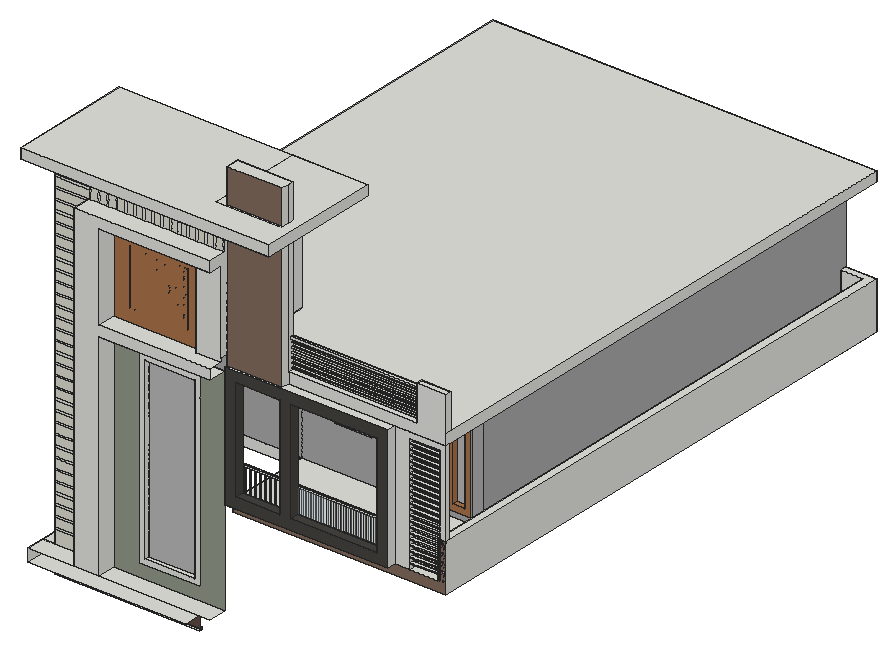
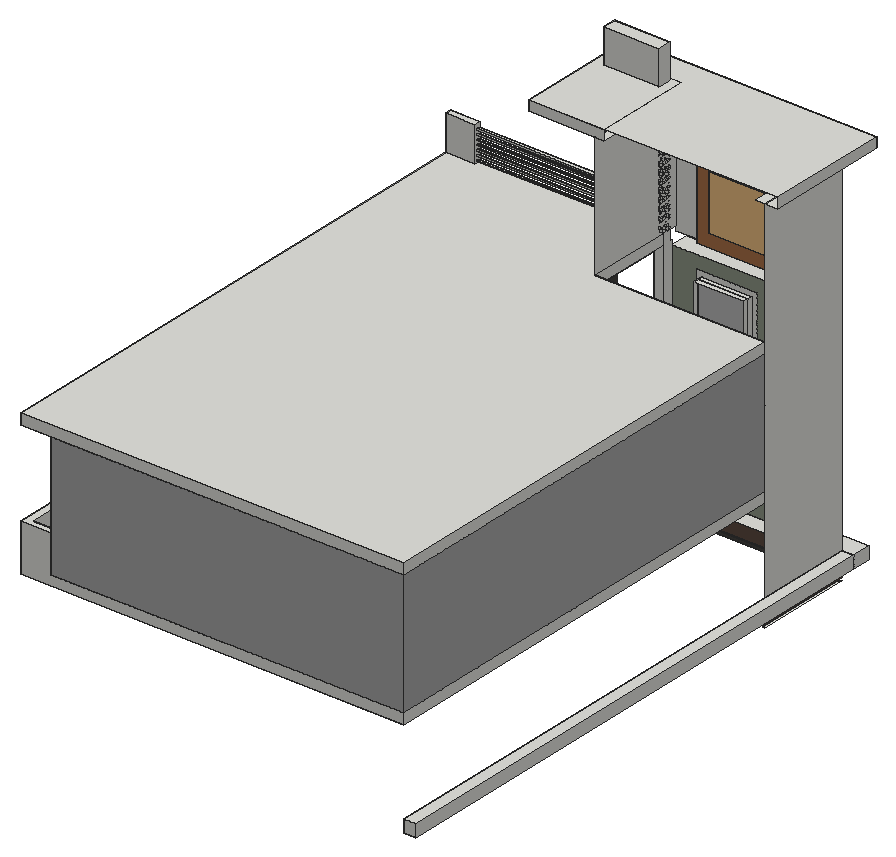
# SketchUp Ruby script. Lengths in inches.
U = 1.inch
M = Sketchup.active_model
def pt(a) = Geom::Point3d.new(a.map { |v| v * U })
def face(e, loops, mat)
  f = e.add_face(loops[0].map { |a| pt(a) })
  loops[1..].each { |l| e.add_face(l.map { |a| pt(a) }).erase! }
  f.material = f.back_material = mat if mat
  f
end
# faces: each face lists its corners as indices into pts; further lists are holes
def faces(e, pts, list, mat = nil) = list.each { |f| face(e, (f[0].is_a?(Array) ? f : [f]).map { |l| l.map { |i| pts[i] } }, mat) }
# xy, xz, yz: faces in a plane at the given z, y or x. An outline is a flat list of corners, or four numbers for a rectangle; further outlines are holes
def ring(l) = l.size == 4 ? [[l[0], l[1]], [l[2], l[1]], [l[2], l[3]], [l[0], l[3]]] : l.each_slice(2).to_a
def flat(e, list, mat, &to3) = list.each { |f| face(e, (f[0].is_a?(Array) ? f : [f]).map { |l| ring(l).map { |u, v| to3.(u, v) } }, mat) }
def xy(e, z, list, mat = nil) = flat(e, list, mat) { |x, y| [x, y, z] }
def xz(e, y, list, mat = nil) = flat(e, list, mat) { |x, z| [x, y, z] }
def yz(e, x, list, mat = nil) = flat(e, list, mat) { |y, z| [x, y, z] }
def lines(e, pts, list) = list.each { |a, b| e.add_line(pt(pts[a]), pt(pts[b])) }
# prism: a flat outline (further loops are holes) pulled along v
def prism(e, loops, v, mat = nil)
  f = face(e, loops, mat); d = Geom::Vector3d.new(v.map { |x| x * U })
  f.pushpull(f.normal.samedirection?(d) ? d.length : -d.length)
end
def box(e, o, s, mat = nil) = prism(e, [[o, [o[0] + s[0], o[1], o[2]], [o[0] + s[0], o[1] + s[1], o[2]], [o[0], o[1] + s[1], o[2]]]], [0, 0, s[2]], mat)
def at(x, y, z, deg = 0) = Geom::Transformation.translation(pt([x, y, z])) * Geom::Transformation.rotation(ORIGIN, Z_AXIS, deg.degrees)
def axes(o, x, y, z) = Geom::Transformation.new([*x, 0, *y, 0, *z, 0, *pt(o).to_a, 1])
def part(name) = M.definitions.add(name)
# library, detail: a bought-in or finely detailed component or shape, given as its bounding box
def library(name, o, s) = part(name).tap { |d| box(d.entities, o, s) }
def detail(e, o, s) = box(e.add_group.entities, o, s)
def put(e, d, t, mat = nil) = e.add_instance(d, t).tap { |i| i.material = mat if mat }
def group(e, t, mat = nil) = e.add_group.tap { |g| g.transformation = t; g.material = mat if mat }.entities
root = M.entities
M.materials.add("Glass_Mirror_01").color = [185, 185, 185]
M.materials.add("Glass_Safety_01").color = [2, 2, 2]
M.materials["Glass_Safety_01"].alpha = 0.62
M.materials.add("Glass_Safety_1").color = [204, 235, 244]
M.materials["Glass_Safety_1"].alpha = 0.25
M.materials.add("Image5").color = [194, 200, 205]
M.materials.add("Image7").color = [145, 153, 137]
M.materials.add("M03_Pewter_Shine").color = [168, 168, 168]
M.materials.add("Metal_06_1K").color = [238, 236, 231]
M.materials.add("Milk_White_Licetto-washable_matte_wall_paint").color = [220, 220, 208]
M.materials.add("Wood_Floor_12_1K").color = [132, 108, 93]
M.materials.add("Wood_Floor_12_1K1").color = [92, 75, 65]
M.materials.add("Wood_Planks_01_1K").color = [69, 67, 63]
M.materials.add("Wood_Veneer_15_1K").color = [170, 114, 74]
c1 = library("ganesh ",[0,0,0],[14.78,0.5,14.79])
xy(root,142.01,[[12,57.125,153,59.125],[12,59.125,14,150.125]])
xy(root,144.01,[[12,57.125,153,59.125],[12,59.125,14,150.125]])
xy(root,156.01,[[0,39.125,153,57.125],[0,57.125,12,588.125]])
xy(root,168.01,[[0,39.125,45,57.125],[69,39.125,177,57.125],[0,57.125,12,588.125]])
xy(root,185.46,[[99.34,57.125,147.79,61.625],[99.34,61.625,147.79,66.125]])
xy(root,292.18,[[226.96,67.38,227.77,67.96]])
xy(root,358.09,[[99.34,57.125,147.79,61.625],[99.34,61.625,147.79,66.125]])
xy(root,376,[[69,39.125,177,57.125]])
xy(root,386,[[69,39.125,177,39.125,177,52.125,153,52.125,153,57.125,69,57.125]])
xy(root,469.49,[[69,39.125,69,57.125,153,57.125,153,52.125,177,52.125,177,39.125]])
xy(root,479.49,[[45,39.125,177,57.125]])
xy(root,510,[[0,30.125,0,57.125,177,57.125,177,150.125,241.26,150.125,241.26,30.125],[0,57.125,12,66.125],[12,57.125,168,66.125],[168,57.125,175,150.125],[175,57.125,177,150.125],
  [0,66.125,12,150.125],[12,66.125,21,150.125]])
xy(root,520,[[0,30.125,241.26,150.125]])
xz(root,30.125,[[0,510,241.26,520]])
xz(root,39.125,[[45,168.01,69,168.01,69,376,177,376,177,386,69,386,69,469.49,177,469.49,177,479.49,45,479.49]])
xz(root,52.125,[[153,386,177,469.49]])
xz(root,57.125,[[0,156.01,12,168.01],[[94.34,180.46,152.79,363.09],[99.34,185.46,147.79,358.09]],[12,181.04,45,183.04],[12,191.26,45,193.26],[12,201.47,45,203.47],
  [12,211.68,45,213.68],[12,221.89,45,223.89],[12,232.1,45,234.1],[12,242.32,45,244.32],[12,252.53,45,254.53],
  [12,262.74,45,264.74],[12,272.95,45,274.95],[12,283.16,45,285.16],[12,293.375,45,295.375],[12,303.59,45,305.59],
  [12,313.8,45,315.8],[12,324.01,45,326.01],[12,334.22,45,336.22],[12,344.4375,45,346.4375],[12,354.65,45,356.65],
  [12,364.86,45,366.86],[12,375.07,45,377.07],[12,385.28,45,387.28],[12,395.5,45,397.5],[12,405.71,45,407.71],
  [12,415.92,45,417.92],[12,426.13,45,428.13],[12,436.34,45,438.34],[12,446.56,45,448.56],[12,456.77,45,458.77],
  [12,466.98,45,468.98],[12,477.19,45,479.19],[45,479.49,47,510],[53.67,479.49,55.67,510],[62.33,479.49,64.34,510],
  [71,479.49,73,510],[79.67,479.49,81.67,510],[88.33,479.49,90.34,510],[97,479.49,99,510],[105.66,479.49,107.67,510],
  [114.33,479.49,116.34,510],[123,479.49,125,510],[131.66,479.49,133.67,510],[140.33,479.49,142.33,510],[149,479.49,151,510],
  [157.66,479.49,159.67,510],[166.33,479.49,168.33,510],[175,479.49,177,510],[12,487.4,45,489.4]])
xz(root,57.125,[[[69,168.01,177,376],[94.34,180.46,152.79,363.09]]],"Image7")
xz(root,57.125,[[12,168.01,45,181.04],[12,183.04,45,191.26],[12,193.26,45,201.47],[12,203.47,45,211.68],[12,213.68,45,221.89],
  [12,223.89,45,232.1],[12,234.1,45,242.32],[12,244.32,45,252.53],[12,254.53,45,262.74],[12,264.74,45,272.95],
  [12,274.95,45,283.16],[12,285.16,45,293.375],[12,295.375,45,303.59],[12,305.59,45,313.8],[12,315.8,45,324.01],
  [12,326.01,45,334.22],[12,336.22,45,344.4375],[12,346.4375,45,354.65],[12,356.65,45,364.86],[12,366.86,45,375.07],
  [12,377.07,45,385.28],[12,387.28,45,395.5],[12,397.5,45,405.71],[12,407.71,45,415.92],[12,417.92,45,426.13],
  [12,428.13,45,436.34],[12,438.34,45,446.56],[12,448.56,45,456.77],[12,458.77,45,466.98],[12,468.98,45,477.19],
  [12,479.19,45,487.4],[47,479.49,53.67,510],[55.67,479.49,62.33,510],[64.34,479.49,71,510],[73,479.49,79.67,510],
  [81.67,479.49,88.33,510],[90.34,479.49,97,510],[99,479.49,105.66,510],[107.67,479.49,114.33,510],[116.34,479.49,123,510],
  [125,479.49,131.66,510],[133.67,479.49,140.33,510],[142.33,479.49,149,510],[151,479.49,157.66,510],[159.67,479.49,166.33,510],
  [168.33,479.49,175,510],[12,489.4,45,510]],"Milk_White_Licetto-washable_matte_wall_paint")
xz(root,57.125,[[12,144.01,153,156.01]],"Wood_Floor_12_1K1")
xz(root,57.125,[[69,386,153,469.49]],"Wood_Veneer_15_1K")
xz(root,59.125,[[14,142.01,153,144.01]],"Wood_Planks_01_1K")
xz(root,61.625,[[99.34,185.46,147.79,358.09]],"Glass_Mirror_01")
xz(root,67.77,[[243.15,266.81,243.85,292.18],[246.4,266.81,247.1,292.18],[249.64,266.81,250.34,292.18],[252.89,266.81,253.59,292.18],[256.13,266.81,256.83,292.18],
  [259.38,266.81,260.08,292.18],[262.625,266.81,263.32,292.18],[267.49,266.81,268.19,292.18],[270.74,266.81,271.4375,292.18],[273.98,266.81,274.68,292.18],
  [277.23,266.81,277.93,292.18],[280.47,266.81,281.17,292.18],[283.72,266.81,284.42,292.18],[286.96,266.81,287.66,292.18],[290.21,266.81,290.91,292.18],
  [293.45,266.81,294.15,292.18],[296.7,266.81,297.4,292.18],[299.94,266.81,300.64,292.18],[303.1875,266.81,303.89,292.18],[306.43,266.81,307.13,292.18],
  [309.68,266.81,310.38,292.18],[312.92,266.81,313.62,292.18],[316.17,266.81,316.87,292.18],[319.41,266.81,320.11,292.18],[322.66,266.81,323.36,292.18]])
xz(root,67.77,[[240.53,266.81,240.61,292.18]],"Glass_Safety_1")
xz(root,150.125,[[168,510,241.26,520]])
xz(root,588.125,[[0,156.01,12,168.01]])
yz(root,0,[[39.125,156.01,57.125,168.01],[57.125,156.01,588.125,168.01],[30.125,510,150.125,520]])
yz(root,12,[[57.125,156.01,150.125,168.01],[150.125,156.01,588.125,168.01],[57.125,168.01,150.125,510]])
yz(root,12,[[57.125,144.01,150.125,156.01]],"Wood_Floor_12_1K1")
yz(root,14,[[59.125,142.01,150.125,144.01]],"Wood_Planks_01_1K")
yz(root,45,[[39.125,168.01,57.125,479.49]])
yz(root,69,[[39.125,168.01,57.125,376],[39.125,386,57.125,469.49]])
yz(root,99.34,[[57.125,185.46,61.625,358.09],[61.625,185.46,66.125,358.09]])
yz(root,147.79,[[57.125,185.46,61.625,358.09],[61.625,185.46,66.125,358.09]])
yz(root,153,[[52.125,386,57.125,469.49]])
yz(root,177,[[52.125,390,150.125,390,150.125,510,57.125,510,57.125,479.49,39.125,479.49,39.125,469.49,52.125,469.49]])
yz(root,241.26,[[30.125,510,150.125,520]])
p = [[334.61,67.85,292.18],[243.85,67.77,292.18],[243.85,67.77,266.81],[243.23,67.77,266.81],[243.15,67.77,266.81],[243.15,67.77,292.18],
  [240.61,67.77,292.18],[240.61,67.77,266.81],[240.53,67.77,266.81],[240.53,67.77,292.18],[240.32,67.77,292.18],[233.65,67.77,292.18],
  [233.65,67.77,262.23],[334.61,67.85,262.23],[240.32,67.77,269.07],[240.32,67.77,266.81],[244.85,67.77,266.81],[245.48,67.77,266.81],
  [245.48,67.77,292.18],[244.78,67.77,292.18],[244.78,67.77,266.81],[248.1,67.77,266.81],[248.72,67.77,266.81],[248.72,67.77,292.18],
  [248.02,67.77,292.18],[248.02,67.77,266.81],[251.34,67.77,266.81],[251.97,67.77,266.81],[251.97,67.77,292.18],[251.27,67.77,292.18],
  [251.27,67.77,266.81],[254.59,67.77,266.81],[255.21,67.77,266.81],[255.21,67.77,292.18],[254.51,67.77,292.18],[254.51,67.77,266.81],
  [257.83,67.77,266.81],[258.46,67.77,266.81],[258.46,67.77,292.18],[257.76,67.77,292.18],[257.76,67.77,266.81],[261.08,67.77,266.81],
  [261.7,67.77,266.81],[261.7,67.77,292.18],[261,67.77,292.18],[261,67.77,266.81],[264.32,67.77,266.81],[264.95,67.77,266.81],
  [264.95,67.77,292.18],[264.25,67.77,292.18],[264.25,67.77,266.81],[265.95,67.77,266.81],[266.57,67.77,266.81],[266.57,67.77,292.18],
  [265.87,67.77,292.18],[265.87,67.77,266.81],[269.19,67.77,266.81],[269.8125,67.77,266.81],[269.8125,67.77,292.18],[269.11,67.77,292.18],
  [269.11,67.77,266.81],[272.4375,67.77,266.81],[273.06,67.77,266.81],[273.06,67.77,292.18],[272.36,67.77,292.18],[272.36,67.77,266.81],
  [275.68,67.77,266.81],[276.3,67.77,266.81],[276.3,67.77,292.18],[275.6,67.77,292.18],[275.6,67.77,266.81],[278.93,67.77,266.81],
  [279.55,67.77,266.81],[279.55,67.77,292.18],[278.85,67.77,292.18],[278.85,67.77,266.81],[282.17,67.77,266.81],[282.79,67.77,266.81],
  [282.79,67.77,292.18],[282.09,67.77,292.18],[282.09,67.77,266.81],[285.42,67.77,266.81],[286.04,67.77,266.81],[286.04,67.77,292.18],
  [285.34,67.77,292.18],[285.34,67.77,266.81],[288.66,67.77,266.81],[289.28,67.77,266.81],[289.28,67.77,292.18],[288.58,67.77,292.18],
  [288.58,67.77,266.81],[291.91,67.77,266.81],[292.53,67.77,266.81],[292.53,67.77,292.18],[291.83,67.77,292.18],[291.83,67.77,266.81],
  [295.15,67.77,266.81],[295.77,67.77,266.81],[295.77,67.77,292.18],[295.07,67.77,292.18],[295.07,67.77,266.81],[298.4,67.77,266.81],
  [299.02,67.77,266.81],[299.02,67.77,292.18],[298.32,67.77,292.18],[298.32,67.77,266.81],[168,57.125,520],[230.05,57.125,520],
  [229.85,72.13,519.8],[230.05,72.13,510],[168,150.125,520]]
faces(root,p,[[0,1,2,3,4,5,6,7,8,9,10,11,12,13]],"Glass_Safety_1")
lines(root,p,[[10,14],[14,15],[16,17],[18,19],[20,16],[21,22],[23,24],[25,21],[26,27],[28,29],[30,26],[31,32],
  [33,34],[35,31],[36,37],[38,39],[40,36],[41,42],[43,44],[45,41],[46,47],[48,49],[50,46],[51,52],
  [53,54],[55,51],[56,57],[58,59],[60,56],[61,62],[63,64],[65,61],[66,67],[68,69],[70,66],[71,72],
  [73,74],[75,71],[76,77],[78,79],[80,76],[81,82],[83,84],[85,81],[86,87],[88,89],[90,86],[91,92],
  [93,94],[95,91],[96,97],[98,99],[100,96],[101,102],[103,104],[105,101],[106,107],[108,109],[106,110]])
g1 = group(root,at(12,150.125,250))
xy(g1,0,[[165,-84,165,0,0,0,0,438,372,438,372,-84]])
xy(g1,10,[[165,-84,363.98,-84,363.98,431.93,342,431.93,342,438,0,438,0,0,165,0]])
xy(g1,46,[[363.98,-84,372,-84,372,438,342,438,342,431.93,363.98,431.93]])
xz(g1,-84,[[165,0,372,0,372,46,363.98,46,363.98,10,165,10]],"Wood_Floor_12_1K")
xz(g1,0,[[0,0,165,10]])
xz(g1,431.93,[[342,10,363.98,46]])
xz(g1,438,[[0,0,0,10,342,10,342,46,372,46,372,0]])
yz(g1,0,[[0,0,438,10]])
yz(g1,165,[[-84,0,0,10]])
yz(g1,342,[[431.93,10,438,46]])
yz(g1,363.98,[[-84,10,431.93,46]])
yz(g1,372,[[-84,0,438,46]])
g2 = group(root,at(12,150.125,260),"M03_Pewter_Shine")
xy(g2,0,[[9,9,333,429]])
xy(g2,6,[[258,-1,330,0]])
xy(g2,12,[[264,4.5,276,9],[281,4.5,307,9],[312,4.5,324,9]])
xy(g2,12,[[264,-1,276,4.5],[281,-1,307,4.5],[312,-1,324,4.5]],"Wood_Veneer_15_1K")
xy(g2,42,[[198,-1,234,0]])
xy(g2,45,[[201,4.5,214.5,9],[217.5,4.5,231,9]])
xy(g2,45,[[201,-1,214.5,4.5],[217.5,-1,231,4.5]],"Wood_Planks_01_1K")
xy(g2,87,[[201,4.5,214.5,9],[217.5,4.5,231,9]])
xy(g2,87,[[201,-1,214.5,4.5],[217.5,-1,231,4.5]],"Wood_Planks_01_1K")
xy(g2,90,[[198,-1,234,0],[264,4.5,276,9],[281,4.5,307,9],[312,4.5,324,9]])
xy(g2,90,[[264,-1,276,4.5],[281,-1,307,4.5],[312,-1,324,4.5]],"Wood_Veneer_15_1K")
xy(g2,96,[[258,-1,330,0]])
xy(g2,120,[[[0,0,342,438],[9,9,333,429]]])
xz(g2,-1,[[[198,42,234,90],[199.48,43.48,232.52,88.52]]])
xz(g2,-1,[[[199.48,43.48,232.52,88.52],[201,45,214.5,87],[217.5,45,231,87]]],"Wood_Planks_01_1K")
xz(g2,-1,[[[258,6,330,96],[281,12,307,90],[264,12,276,90],[312,12,324,90]]],"Wood_Veneer_15_1K")
xz(g2,0,[[0,0,9,120],[9,0,156,120],[156,0,165,120],[[165,0,342,120],[258,6,330,96],[198,42,234,90]]])
xz(g2,4.5,[[264,12,276,90],[281,12,307,90],[312,12,324,90]],"Glass_Mirror_01")
xz(g2,4.5,[[201,45,214.5,87],[217.5,45,231,87]],"Glass_Safety_01")
xz(g2,9,[[[9,0,333,120],[281,12,307,90],[264,12,276,90],[312,12,324,90],[201,45,214.5,87],[217.5,45,231,87]]])
xz(g2,429,[[9,0,333,120]])
xz(g2,438,[[0,0,342,120]])
yz(g2,0,[[0,0,438,120]])
yz(g2,9,[[9,0,429,120]])
yz(g2,198,[[-1,42,0,90]])
yz(g2,201,[[4.5,45,9,87]])
yz(g2,201,[[-1,45,4.5,87]],"Wood_Planks_01_1K")
yz(g2,214.5,[[4.5,45,9,87]])
yz(g2,214.5,[[-1,45,4.5,87]],"Wood_Planks_01_1K")
yz(g2,217.5,[[4.5,45,9,87]])
yz(g2,217.5,[[-1,45,4.5,87]],"Wood_Planks_01_1K")
yz(g2,231,[[4.5,45,9,87]])
yz(g2,231,[[-1,45,4.5,87]],"Wood_Planks_01_1K")
yz(g2,234,[[-1,42,0,90]])
yz(g2,258,[[-1,6,0,96]])
yz(g2,264,[[4.5,12,9,90]])
yz(g2,264,[[-1,12,4.5,90]],"Wood_Veneer_15_1K")
yz(g2,276,[[4.5,12,9,90]])
yz(g2,276,[[-1,12,4.5,90]],"Wood_Veneer_15_1K")
yz(g2,281,[[4.5,12,9,90]])
yz(g2,281,[[-1,12,4.5,90]],"Wood_Veneer_15_1K")
yz(g2,307,[[4.5,12,9,90]])
yz(g2,307,[[-1,12,4.5,90]],"Wood_Veneer_15_1K")
yz(g2,312,[[4.5,12,9,90]])
yz(g2,312,[[-1,12,4.5,90]],"Wood_Veneer_15_1K")
yz(g2,324,[[4.5,12,9,90]])
yz(g2,324,[[-1,12,4.5,90]],"Wood_Veneer_15_1K")
yz(g2,330,[[-1,6,0,96]])
yz(g2,333,[[9,0,429,120]])
yz(g2,342,[[0,0,438,120]])
g3 = group(root,at(12,150.125,380))
xy(g3,-120,[[165,-93,322.61,-84],[322.61,-84,337.23,-80.37],[366,-84,372,-80.37]])
xy(g3,-119.18,[[175.87,-82.74,176.68,-82.16],[180.75,-82.74,181.5625,-82.16],[185.64,-82.74,186.45,-82.16],[190.53,-82.74,191.34,-82.16],[195.41,-82.74,196.22,-82.16],
  [200.3,-82.74,201.11,-82.16],[205.1875,-82.74,206,-82.16],[210.07,-82.74,210.88,-82.16],[214.96,-82.74,215.77,-82.16]])
xy(g3,-114.78,[[337.23,-84,366,-80.37]])
xy(g3,-113.78,[[337.23,-84,366,-80.37]])
xy(g3,-110,[[175,-93,218.35,-84],[228.35,-93,312.61,-84]],"Wood_Planks_01_1K")
xy(g3,-109.59,[[337.23,-84,366,-80.37]])
xy(g3,-108.59,[[337.23,-84,366,-80.37]])
xy(g3,-104.4,[[337.23,-84,366,-80.37]])
xy(g3,-103.4,[[337.23,-84,366,-80.37]])
xy(g3,-99.22,[[337.23,-84,366,-80.37]])
xy(g3,-98.22,[[337.23,-84,366,-80.37]])
xy(g3,-94.03,[[337.23,-84,366,-80.37]])
xy(g3,-93.03,[[337.23,-84,366,-80.37]])
xy(g3,-88.84,[[337.23,-84,366,-80.37]])
xy(g3,-87.84,[[337.23,-84,366,-80.37]])
xy(g3,-87.82,[[[154.27,-83.0625,322.61,-81.79],[214.96,-82.74,215.77,-82.16],[210.07,-82.74,210.88,-82.16],[205.1875,-82.74,206,-82.16],[200.3,-82.74,201.11,-82.16],[195.41,-82.74,196.22,-82.16],[190.53,-82.74,191.34,-82.16],[185.64,-82.74,186.45,-82.16],[180.75,-82.74,181.5625,-82.16],[175.87,-82.74,176.68,-82.16]]])
xy(g3,-85.42,[[154.27,-83.0625,322.61,-81.79]])
xy(g3,-83.65,[[337.23,-84,366,-80.37]])
xy(g3,-82.65,[[337.23,-84,366,-80.37]])
xy(g3,-78.46,[[337.23,-84,366,-80.37]])
xy(g3,-77.46,[[337.23,-84,366,-80.37]])
xy(g3,-73.27,[[337.23,-84,366,-80.37]])
xy(g3,-72.27,[[337.23,-84,366,-80.37]])
xy(g3,-68.08,[[337.23,-84,366,-80.37]])
xy(g3,-67.08,[[337.23,-84,366,-80.37]])
xy(g3,-62.89,[[337.23,-84,366,-80.37]])
xy(g3,-61.89,[[337.23,-84,366,-80.37]])
xy(g3,-57.7,[[337.23,-84,366,-80.37]])
xy(g3,-56.7,[[337.23,-84,366,-80.37]])
xy(g3,-52.51,[[337.23,-84,366,-80.37]])
xy(g3,-51.51,[[337.23,-84,366,-80.37]])
xy(g3,-47.32,[[337.23,-84,366,-80.37]])
xy(g3,-46.32,[[337.23,-84,366,-80.37]])
xy(g3,-42.13,[[337.23,-84,366,-80.37]])
xy(g3,-41.13,[[337.23,-84,366,-80.37]])
xy(g3,-36.95,[[337.23,-84,366,-80.37]])
xy(g3,-35.95,[[337.23,-84,366,-80.37]])
xy(g3,-31.76,[[337.23,-84,366,-80.37]])
xy(g3,-30.76,[[337.23,-84,366,-80.37]])
xy(g3,-26.57,[[337.23,-84,366,-80.37]])
xy(g3,-25.57,[[337.23,-84,366,-80.37]])
xy(g3,-21.38,[[337.23,-84,366,-80.37]])
xy(g3,-20.38,[[337.23,-84,366,-80.37]])
xy(g3,-16.1875,[[337.23,-84,366,-80.37]])
xy(g3,-15.1875,[[337.23,-84,366,-80.37]])
xy(g3,-11,[[337.23,-84,366,-80.37]])
xy(g3,-10,[[312.61,-84,322.61,0],[337.23,-84,366,-80.37]])
xy(g3,-10,[[175,-93,175,0,312.61,0,312.61,-93,228.35,-93,228.35,-84,218.35,-84,218.35,-93]],"Image5")
xy(g3,-6,[[337.23,-84,366,-80.37]])
xy(g3,0,[[165,-93,218.53,-93,218.6875,-90.87,165,-90.87],[218.53,-93,322.61,-93,322.61,-84,219.19,-84,218.6875,-90.87],[165,-84,165,0,0,0,0,438,372,438,372,-80.37,322.61,-80.37,322.61,0,175,0,175,-84],[175,-84,312.61,0],[312.61,-84,322.61,0],
  [322.61,-84,372,-80.37]])
xy(g3,10,[[219.19,-84,343.57,-84,343.57,-78.05,371.96,-78.05,371.96,-84,372,-84,372,438,0,438,0,0,165,0,165,-77.99,219.19,-77.99],[165,-84,175,-77.99],[175,-84,219.19,-77.99]])
xy(g3,12,[[219.19,-80.65,343.57,-79.24]])
xy(g3,13.27,[[219.19,-80.65,343.57,-79.24]])
xy(g3,16.54,[[219.19,-80.65,343.57,-79.24]])
xy(g3,17.8125,[[219.19,-80.65,343.57,-79.24]])
xy(g3,21.09,[[219.19,-80.65,343.57,-79.24]])
xy(g3,22.36,[[219.19,-80.65,343.57,-79.24]])
xy(g3,25.625,[[219.19,-80.65,343.57,-79.24]])
xy(g3,26.9,[[219.19,-80.65,343.57,-79.24]])
xy(g3,30.17,[[219.19,-80.65,343.57,-79.24]])
xy(g3,31.4375,[[219.19,-80.65,343.57,-79.24]])
xy(g3,34.71,[[219.19,-80.65,343.57,-79.24]])
xy(g3,35.98,[[219.19,-80.65,343.57,-79.24]])
xy(g3,38.65,[[219.19,-82.17,343.57,-79.1]])
xy(g3,40.52,[[219.19,-82.17,343.57,-79.1]])
xy(g3,44.18,[[343.57,-84,371.96,-78.05]])
xy(g3,172.88,[[165,-90.87,218.6875,-90.87,219.19,-84,219.19,-77.99,165,-77.99]])
xz(g3,-93,[[[165,-120,322.61,0],[228.35,-110,312.61,-10],[175,-110,218.35,-10]]],"Wood_Planks_01_1K")
xz(g3,-90.87,[[165,0,218.6875,172.88]],"Wood_Floor_12_1K")
xz(g3,-84,[[165,-120,165,0,175,0,175,-110,218.35,-110,218.35,-10,228.35,-10,228.35,-110,312.61,-110,312.61,-10,322.61,-10,322.61,-120],[322.61,-120,337.23,-120,337.23,-6,366,-6,366,-120,372,-120,372,0,322.61,0],[337.23,-114.78,366,-113.78],[337.23,-109.59,366,-108.59],[337.23,-104.4,366,-103.4],
  [337.23,-99.22,366,-98.22],[337.23,-94.03,366,-93.03],[337.23,-88.84,366,-87.84],[337.23,-83.65,366,-82.65],[337.23,-78.46,366,-77.46],
  [337.23,-73.27,366,-72.27],[337.23,-68.08,366,-67.08],[337.23,-62.89,366,-61.89],[337.23,-57.7,366,-56.7],[337.23,-52.51,366,-51.51],
  [337.23,-47.32,366,-46.32],[337.23,-42.13,366,-41.13],[337.23,-36.95,366,-35.95],[337.23,-31.76,366,-30.76],[337.23,-26.57,366,-25.57],
  [337.23,-21.38,366,-20.38],[337.23,-16.1875,366,-15.1875],[337.23,-11,366,-10],[165,0,175,10],[175,0,219.19,10],
  [219.19,0,372,0,372,10,371.96,10,371.96,44.18,343.57,44.18,343.57,10,219.19,10]])
xz(g3,-83.0625,[[154.27,-87.82,322.61,-85.42]],"Metal_06_1K")
xz(g3,-82.74,[[175.87,-119.18,176.68,-87.82],[180.75,-119.18,181.5625,-87.82],[185.64,-119.18,186.45,-87.82],[190.53,-119.18,191.34,-87.82],[195.41,-119.18,196.22,-87.82],
  [200.3,-119.18,201.11,-87.82],[205.1875,-119.18,206,-87.82],[210.07,-119.18,210.88,-87.82],[214.96,-119.18,215.77,-87.82]],"Metal_06_1K")
xz(g3,-82.17,[[219.19,38.65,343.57,40.52]])
xz(g3,-82.16,[[175.87,-119.18,176.68,-87.82],[180.75,-119.18,181.5625,-87.82],[185.64,-119.18,186.45,-87.82],[190.53,-119.18,191.34,-87.82],[195.41,-119.18,196.22,-87.82],
  [200.3,-119.18,201.11,-87.82],[205.1875,-119.18,206,-87.82],[210.07,-119.18,210.88,-87.82],[214.96,-119.18,215.77,-87.82]],"Metal_06_1K")
xz(g3,-81.79,[[154.27,-87.82,322.61,-85.42]])
xz(g3,-80.65,[[219.19,12,343.57,13.27],[219.19,16.54,343.57,17.8125],[219.19,21.09,343.57,22.36],[219.19,25.625,343.57,26.9],[219.19,30.17,343.57,31.4375],
  [219.19,34.71,343.57,35.98]])
xz(g3,-80.37,[[[322.61,-120,322.61,0,372,0,372,-84,366,-84,366,-83.65,337.23,-83.65,337.23,-87.84,366,-87.84,366,-88.84,337.23,-88.84,337.23,-93.03,366,-93.03,366,-94.03,337.23,-94.03,337.23,-98.22,366,-98.22,366,-99.22,337.23,-99.22,337.23,-103.4,366,-103.4,366,-104.4,337.23,-104.4,337.23,-108.59,366,-108.59,366,-109.59,337.23,-109.59,337.23,-113.78,366,-113.78,366,-114.78,337.23,-114.78,337.23,-120],[337.23,-20.38,366,-16.1875],[337.23,-30.76,366,-26.57],[337.23,-41.13,366,-36.95],[337.23,-51.51,366,-47.32],[337.23,-61.89,366,-57.7],[337.23,-72.27,366,-68.08],[337.23,-15.1875,366,-11],[337.23,-25.57,366,-21.38],[337.23,-35.95,366,-31.76],[337.23,-46.32,366,-42.13],[337.23,-56.7,366,-52.51],[337.23,-67.08,366,-62.89],[337.23,-77.46,366,-73.27],[337.23,-82.65,366,-78.46],[337.23,-10,366,-6]],[366,-120,372,-84]])
xz(g3,-79.24,[[219.19,12,343.57,13.27],[219.19,16.54,343.57,17.8125],[219.19,21.09,343.57,22.36],[219.19,25.625,343.57,26.9],[219.19,30.17,343.57,31.4375],
  [219.19,34.71,343.57,35.98]])
xz(g3,-79.1,[[219.19,38.65,343.57,40.52]])
xz(g3,-78.05,[[343.57,10,371.96,44.18]])
xz(g3,-77.99,[[165,10,219.19,172.88]])
xz(g3,0,[[175,-10,322.61,0],[0,0,165,10]])
xz(g3,438,[[0,0,372,10]])
yz(g3,0,[[0,0,438,10]])
yz(g3,154.27,[[-83.0625,-87.82,-81.79,-85.42]])
yz(g3,165,[[-93,-120,-93,0,-90.87,0,-90.87,172.88,-77.99,172.88,-77.99,10,-84,10,-84,-120],[-84,0,0,10]])
yz(g3,175,[[-84,-10,0,0]])
yz(g3,175,[[-93,-110,-84,-10]],"Wood_Planks_01_1K")
yz(g3,175.87,[[-82.74,-119.18,-82.16,-87.82]])
yz(g3,176.68,[[-82.74,-119.18,-82.16,-87.82]])
yz(g3,180.75,[[-82.74,-119.18,-82.16,-87.82]])
yz(g3,181.5625,[[-82.74,-119.18,-82.16,-87.82]])
yz(g3,185.64,[[-82.74,-119.18,-82.16,-87.82]])
yz(g3,186.45,[[-82.74,-119.18,-82.16,-87.82]])
yz(g3,190.53,[[-82.74,-119.18,-82.16,-87.82]])
yz(g3,191.34,[[-82.74,-119.18,-82.16,-87.82]])
yz(g3,195.41,[[-82.74,-119.18,-82.16,-87.82]])
yz(g3,196.22,[[-82.74,-119.18,-82.16,-87.82]])
yz(g3,200.3,[[-82.74,-119.18,-82.16,-87.82]])
yz(g3,201.11,[[-82.74,-119.18,-82.16,-87.82]])
yz(g3,205.1875,[[-82.74,-119.18,-82.16,-87.82]],"Metal_06_1K")
yz(g3,206,[[-82.74,-119.18,-82.16,-87.82]])
yz(g3,210.07,[[-82.74,-119.18,-82.16,-87.82]],"Metal_06_1K")
yz(g3,210.88,[[-82.74,-119.18,-82.16,-87.82]],"Metal_06_1K")
yz(g3,214.96,[[-82.74,-119.18,-82.16,-87.82]],"Metal_06_1K")
yz(g3,215.77,[[-82.74,-119.18,-82.16,-87.82]])
yz(g3,218.35,[[-93,-110,-84,-10]],"Wood_Planks_01_1K")
yz(g3,219.19,[[[-84,10,-77.99,172.88],[-82.17,38.65,-79.1,40.52],[-80.65,34.71,-79.24,35.98]]])
yz(g3,228.35,[[-93,-110,-84,-10]],"Wood_Planks_01_1K")
yz(g3,312.61,[[-93,-110,-84,-10]],"Wood_Planks_01_1K")
yz(g3,322.61,[[-93,-120,-84,0],[[-84,-120,-80.37,-10],[-83.0625,-87.82,-81.79,-85.42]],[-84,-10,-80.37,0],[-80.37,-10,0,0]])
yz(g3,337.23,[[-84,-120,-80.37,-114.78],[-84,-113.78,-80.37,-109.59],[-84,-108.59,-80.37,-104.4],[-84,-103.4,-80.37,-99.22],[-84,-98.22,-80.37,-94.03],
  [-84,-93.03,-80.37,-88.84],[-84,-87.84,-80.37,-83.65],[-84,-82.65,-80.37,-78.46],[-84,-77.46,-80.37,-73.27],[-84,-72.27,-80.37,-68.08],
  [-84,-67.08,-80.37,-62.89],[-84,-61.89,-80.37,-57.7],[-84,-56.7,-80.37,-52.51],[-84,-51.51,-80.37,-47.32],[-84,-46.32,-80.37,-42.13],
  [-84,-41.13,-80.37,-36.95],[-84,-35.95,-80.37,-31.76],[-84,-30.76,-80.37,-26.57],[-84,-25.57,-80.37,-21.38],[-84,-20.38,-80.37,-16.1875],
  [-84,-15.1875,-80.37,-11],[-84,-10,-80.37,-6]])
yz(g3,343.57,[[[-84,10,-78.05,44.18],[-82.17,38.65,-79.1,40.52],[-80.65,34.71,-79.24,35.98]]])
yz(g3,366,[[-84,-120,-80.37,-114.78],[-84,-114.78,-80.37,-113.78],[-84,-113.78,-80.37,-109.59],[-84,-109.59,-80.37,-108.59],[-84,-108.59,-80.37,-104.4],
  [-84,-104.4,-80.37,-103.4],[-84,-103.4,-80.37,-99.22],[-84,-99.22,-80.37,-98.22],[-84,-98.22,-80.37,-94.03],[-84,-94.03,-80.37,-93.03],
  [-84,-93.03,-80.37,-88.84],[-84,-88.84,-80.37,-87.84],[-84,-87.84,-80.37,-83.65],[-84,-82.65,-80.37,-78.46],[-84,-77.46,-80.37,-73.27],
  [-84,-72.27,-80.37,-68.08],[-84,-67.08,-80.37,-62.89],[-84,-61.89,-80.37,-57.7],[-84,-56.7,-80.37,-52.51],[-84,-51.51,-80.37,-47.32],
  [-84,-46.32,-80.37,-42.13],[-84,-41.13,-80.37,-36.95],[-84,-35.95,-80.37,-31.76],[-84,-30.76,-80.37,-26.57],[-84,-25.57,-80.37,-21.38],
  [-84,-20.38,-80.37,-16.1875],[-84,-15.1875,-80.37,-11],[-84,-10,-80.37,-6]])
yz(g3,371.96,[[-84,10,-78.05,44.18]])
yz(g3,372,[[-84,-120,-80.37,0],[-84,0,438,10]])
p = [[218.6875,-90.87,0],[219.19,-84,0],[219.19,-84,10],[219.19,-84,172.88],[218.6875,-90.87,172.88]]
faces(g3,p,[[0,1,2,3,4]])
put(root,c1,axes([84.78,57.125,398.83],[3.78835,0,0],[0,1,0],[0,0,3.61681]),"Metal_06_1K")
